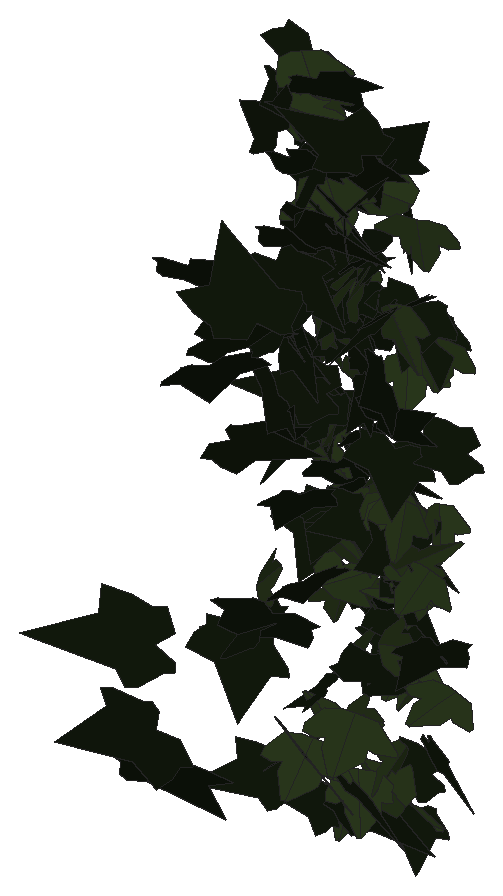
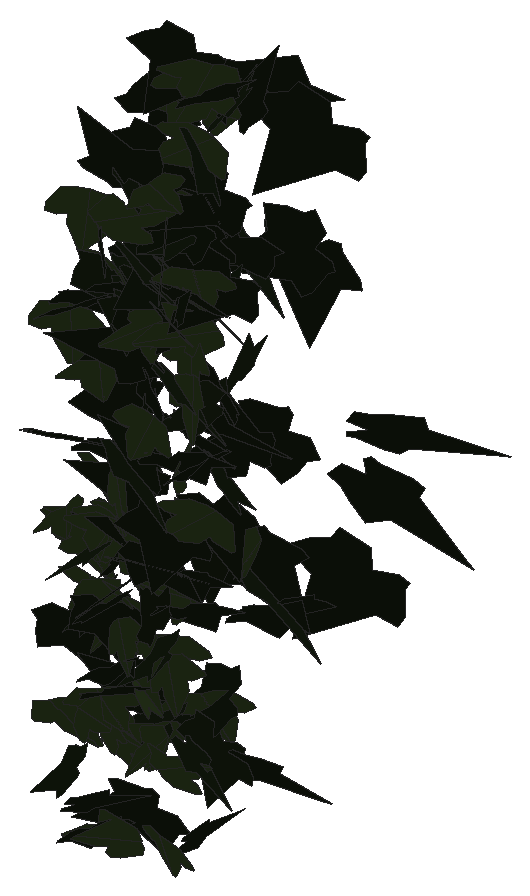
# SketchUp Ruby script. Lengths in inches.
U = 1.inch
M = Sketchup.active_model
def pt(a) = Geom::Point3d.new(a.map { |v| v * U })
def face(e, loops, mat)
  f = e.add_face(loops[0].map { |a| pt(a) })
  loops[1..].each { |l| e.add_face(l.map { |a| pt(a) }).erase! }
  f.material = f.back_material = mat if mat
  f
end
# faces: each face lists its corners as indices into pts; further lists are holes
def faces(e, pts, list, mat = nil) = list.each { |f| face(e, (f[0].is_a?(Array) ? f : [f]).map { |l| l.map { |i| pts[i] } }, mat) }
# xy, xz, yz: faces in a plane at the given z, y or x. An outline is a flat list of corners, or four numbers for a rectangle; further outlines are holes
def ring(l) = l.size == 4 ? [[l[0], l[1]], [l[2], l[1]], [l[2], l[3]], [l[0], l[3]]] : l.each_slice(2).to_a
def flat(e, list, mat, &to3) = list.each { |f| face(e, (f[0].is_a?(Array) ? f : [f]).map { |l| ring(l).map { |u, v| to3.(u, v) } }, mat) }
def xy(e, z, list, mat = nil) = flat(e, list, mat) { |x, y| [x, y, z] }
def xz(e, y, list, mat = nil) = flat(e, list, mat) { |x, z| [x, y, z] }
def yz(e, x, list, mat = nil) = flat(e, list, mat) { |y, z| [x, y, z] }
def lines(e, pts, list) = list.each { |a, b| e.add_line(pt(pts[a]), pt(pts[b])) }
# prism: a flat outline (further loops are holes) pulled along v
def prism(e, loops, v, mat = nil)
  f = face(e, loops, mat); d = Geom::Vector3d.new(v.map { |x| x * U })
  f.pushpull(f.normal.samedirection?(d) ? d.length : -d.length)
end
def box(e, o, s, mat = nil) = prism(e, [[o, [o[0] + s[0], o[1], o[2]], [o[0] + s[0], o[1] + s[1], o[2]], [o[0], o[1] + s[1], o[2]]]], [0, 0, s[2]], mat)
def at(x, y, z, deg = 0) = Geom::Transformation.translation(pt([x, y, z])) * Geom::Transformation.rotation(ORIGIN, Z_AXIS, deg.degrees)
def axes(o, x, y, z) = Geom::Transformation.new([*x, 0, *y, 0, *z, 0, *pt(o).to_a, 1])
def part(name) = M.definitions.add(name)
# library, detail: a bought-in or finely detailed component or shape, given as its bounding box
def library(name, o, s) = part(name).tap { |d| box(d.entities, o, s) }
def detail(e, o, s) = box(e.add_group.entities, o, s)
def put(e, d, t, mat = nil) = e.add_instance(d, t).tap { |i| i.material = mat if mat }
def group(e, t, mat = nil) = e.add_group.tap { |g| g.transformation = t; g.material = mat if mat }.entities
root = M.entities
M.materials.add("1026 AP 7946 SUNNY SIDE UP").color = [254, 231, 186]
M.materials.add("efeu1").color = [18, 25, 13]
M.materials.add("efeu2").color = [43, 57, 29]
c1 = part("ivyleaf_9")
p = [[1.54,2.16,1.25],[1.36,2.04,1.19],[-0.21,0.99,0.68],[-0.71,1.11,0.82],[-0.85,0.86,0.67],[-0.8,0.17,0.21],
  [-0.9,-0.01,0.1],[-0.67,-0.16,-0.02],[-0.08,-0.08,-0.05],[-0.03,-0.6,-0.4],[0.65,-0.88,-0.66],[0.83,-0.6,-0.49],
  [1.29,-0.42,-0.43],[1.8125,-0.07,-0.26],[1.21,0.44,0.15]]
faces(c1.entities,p,[[0,1,2,3,4,5,6,7,8,9,10,11,12,13,14]],"efeu1")
c2 = part("ivyleaf_10")
p = [[0,0.5,-0.03],[-0.0625,2.02,-0.43],[-0.19,2.01,-0.46],[-0.54,1.05,-0.29],[-0.52,0.625,-0.18],[-0.83,0.76,-0.28],
  [-1.16,0.64,-0.33],[-1.15,0.33,-0.24],[-0.77,-0.39,0.02],[-0.3,-0.51,0.16],[0.04,-0.48,0.23],[-0.02,2.01,-0.4375],
  [-0.06,2.01,-0.43],[0.04,-0.49,0.23],[0.67,-0.49,0.14],[1.38,0.36,-0.2],[1.375,0.51,-0.24],[0.81,0.65,-0.19],
  [0.62,0.59,-0.15],[0.6,1.09,-0.28],[0.5,1.23,-0.31]]
faces(c2.entities,p,[[0,1,2,3,4,5,6,7,8,9,10],[11,12,0,13,14,15,16,17,18,19,20]],"efeu2")
put(root,c1,axes([99.1,206.72,271.15],[0.04498,-0.045,-0.44132],[-0.62641,-0.18973,-0.00588],[-0.31896,0.36627,-0.0507]),"1026 AP 7946 SUNNY SIDE UP")
put(root,c1,axes([98.72,207.14,272.19],[-0.51404,0.00428,0.31035],[-0.47955,-0.09831,-0.31579],[0.11029,-0.40748,0.07343]),"1026 AP 7946 SUNNY SIDE UP")
put(root,c1,axes([98.68,207.3,270.18],[0.62161,0.16981,0.02208],[0.03504,-0.00076,-0.43202],[-0.28782,0.36664,-0.00491]),"1026 AP 7946 SUNNY SIDE UP")
put(root,c1,axes([99.86,208,277.3],[-0.67057,-0.05266,0.05626],[0.08156,0.04104,0.42566],[-0.09751,0.39648,-0.0309]),"1026 AP 7946 SUNNY SIDE UP")
put(root,c1,axes([98.4,208.48,277.38],[0.62553,0.17776,0.01998],[0.00654,0.02957,-0.43677],[-0.30296,0.36766,0.03183]),"1026 AP 7946 SUNNY SIDE UP")
put(root,c1,axes([98.43,208.82,275.68],[0.21095,0.37186,-0.04905],[-0.00893,-0.05164,-0.42029],[-0.63702,0.12386,-0.01035]),"1026 AP 7946 SUNNY SIDE UP")
put(root,c1,axes([98.19,209.1,275.91],[0.26985,0.1776,0.31427],[0.39467,0.17871,-0.25004],[-0.42373,0.27956,-0.03275]),"1026 AP 7946 SUNNY SIDE UP")
put(root,c1,axes([98.26,209.78,270.9],[-0.23911,-0.32946,-0.03354],[0.02786,0.02238,-0.38322],[0.56046,-0.14167,0.00474]),"1026 AP 7946 SUNNY SIDE UP")
put(root,c1,axes([98.8,209.67,271.57],[0.1294,0.20948,-0.29899],[-0.33012,-0.21517,-0.23039],[-0.49665,0.1976,0.07524]),"1026 AP 7946 SUNNY SIDE UP")
put(root,c1,axes([99.0625,209.6,276.07],[-0.19036,0.33239,0.11651],[-0.11152,0.08763,-0.37268],[-0.58086,-0.12576,0.03337]),"1026 AP 7946 SUNNY SIDE UP")
put(root,c1,axes([98.55,209.71,271.21],[-0.25067,0.32293,0.10148],[-0.12965,0.064,-0.37665],[-0.55438,-0.16098,0.0422]),"1026 AP 7946 SUNNY SIDE UP")
put(root,c2,axes([99.11,210.09,269.35],[0.4743,0.17614,-0.11601],[-0.12369,-0.0907,-0.35278],[-0.33075,0.28651,-0.03444]),"1026 AP 7946 SUNNY SIDE UP")
put(root,c1,axes([98.78,210.1,269.5],[0.44673,-0.23331,0.02396],[0.00637,-0.034,-0.37619],[0.39834,0.26219,-0.02085]),"1026 AP 7946 SUNNY SIDE UP")
put(root,c2,axes([99.82,210.13,269.97],[0.5272,0.14044,-0.07078],[-0.08561,-0.05286,-0.3645],[-0.25062,0.31349,-0.02437]),"1026 AP 7946 SUNNY SIDE UP")
put(root,c1,axes([98.36,210.375,274.52],[-0.04042,-0.1888,0.29806],[-0.03485,-0.28024,-0.20745],[0.57344,-0.03034,0.0084]),"1026 AP 7946 SUNNY SIDE UP")
put(root,c1,axes([98.49,210.2,268.7],[-0.45262,0.01417,0.14584],[-0.23217,-0.02444,-0.2846],[-0.00247,-0.29833,0.02604]),"1026 AP 7946 SUNNY SIDE UP")
put(root,c2,axes([98.46,209.97,271.8],[0.00956,0.03184,0.33715],[-0.21543,0.28833,-0.02479],[-0.49148,-0.12576,0.01742]),"1026 AP 7946 SUNNY SIDE UP")
put(root,c1,axes([99.05,210.11,271.97],[0.10991,0.33158,0.01218],[0.01766,0.00516,-0.36148],[-0.56272,0.06492,-0.00897]),"1026 AP 7946 SUNNY SIDE UP")
put(root,c1,axes([99.53,210.38,269.03],[0.32232,-0.271,0.0525],[0.0718,-0.03449,-0.35439],[0.46308,0.19397,0.01841]),"1026 AP 7946 SUNNY SIDE UP")
put(root,c1,axes([97.84,210.08,273.76],[0.0256,0.11118,-0.34798],[0.08528,0.32261,0.1246],[0.57924,-0.05241,-0.00297]),"1026 AP 7946 SUNNY SIDE UP")
put(root,c1,axes([98.19,210.56,278.54],[0.06125,0.07775,0.34816],[-0.34612,-0.25285,0.08568],[0.44776,-0.20609,0.01861]),"1026 AP 7946 SUNNY SIDE UP")
put(root,c1,axes([100.32,210.25,275.47],[0.16746,-0.06043,-0.37018],[-0.57964,0.06314,-0.11549],[0.13226,0.35321,-0.03745]),"1026 AP 7946 SUNNY SIDE UP")
put(root,c1,axes([98.41,210.67,275.67],[0.00896,-0.15643,0.2996],[0.01816,-0.28169,-0.1715],[0.54696,0.01192,0.00078]),"1026 AP 7946 SUNNY SIDE UP")
put(root,c1,axes([98.37,210.4,276.58],[-0.09156,-0.13299,-0.32269],[0.25238,0.26077,-0.14889],[0.49606,-0.15722,0.01619]),"1026 AP 7946 SUNNY SIDE UP")
put(root,c2,axes([99.7,210.49,268.87],[0.35392,0.26024,-0.02808],[-0.00632,-0.03491,-0.35691],[-0.44458,0.20767,-0.01728]),"1026 AP 7946 SUNNY SIDE UP")
put(root,c1,axes([98.02,210.59,273.54],[0.2746,0.20994,0.14676],[-0.16858,-0.09261,0.28166],[0.38808,-0.18879,0.01851]),"1026 AP 7946 SUNNY SIDE UP")
put(root,c1,axes([98.625,210.375,269.02],[0.12062,0.28903,0.15336],[0.02741,0.13946,-0.31624],[-0.54409,0.0711,0.01807]),"1026 AP 7946 SUNNY SIDE UP")
put(root,c1,axes([98.05,211.02,278.8],[0.21454,-0.21796,-0.18751],[0.1745,-0.13919,0.26726],[-0.43818,-0.16215,0.01462]),"1026 AP 7946 SUNNY SIDE UP")
put(root,c2,axes([100.21,210.7,268.75],[0.19479,0.04618,0.30215],[-0.4715,0.08782,0.10697],[-0.11132,-0.29115,0.07565]),"1026 AP 7946 SUNNY SIDE UP")
put(root,c2,axes([99.95,211.01,269.17],[0.00722,-0.19655,0.24201],[0.07715,-0.22561,-0.21171],[0.50596,0.03721,0.02883]),"1026 AP 7946 SUNNY SIDE UP")
put(root,c1,axes([99.29,210.97,278.39],[-0.01809,0.0418,0.35658],[-0.5476,-0.0915,-0.00003],[0.15428,-0.31986,0.0417]),"1026 AP 7946 SUNNY SIDE UP")
put(root,c1,axes([98.4,210.82,272.77],[0.09272,0.24876,-0.13909],[-0.05593,-0.12909,-0.27443],[-0.47571,0.06366,0.00515]),"1026 AP 7946 SUNNY SIDE UP")
put(root,c1,axes([98.58,211.12,267.93],[0.02459,-0.21937,-0.16423],[0.07449,-0.14673,0.23138],[-0.44546,-0.03665,0.02963]),"1026 AP 7946 SUNNY SIDE UP")
put(root,c2,axes([98.32,210.88,278.77],[-0.09064,-0.09013,-0.29943],[0.46977,0.07677,-0.08233],[0.16203,-0.273,0.07118]),"1026 AP 7946 SUNNY SIDE UP")
put(root,c1,axes([98.13,211.12,273.54],[-0.32686,0.06498,-0.19825],[0.24268,-0.13294,-0.20998],[-0.23021,-0.2324,0.06013]),"1026 AP 7946 SUNNY SIDE UP")
put(root,c1,axes([98.72,210.85,279.37],[0.43159,0.19588,0.01881],[0.04183,-0.00743,-0.34298],[-0.33087,0.25458,-0.01882]),"1026 AP 7946 SUNNY SIDE UP")
put(root,c1,axes([99.61,211.18,275.9],[-0.36839,0.11376,-0.23066],[0.21062,-0.19885,-0.24729],[-0.35853,-0.2337,0.09173]),"1026 AP 7946 SUNNY SIDE UP")
put(root,c2,axes([98.5,211.03,279.06],[-0.46876,-0.11639,-0.10945],[0.17487,0.01394,-0.31944],[0.19413,-0.2936,0.02347]),"1026 AP 7946 SUNNY SIDE UP")
put(root,c1,axes([98.21,211.03,276.89],[0.42067,-0.03492,0.20078],[0.30703,-0.05702,-0.26738],[0.1053,0.30578,-0.02246]),"1026 AP 7946 SUNNY SIDE UP")
put(root,c2,axes([99.9,211.15,272.89],[0.4863,-0.10978,0.07249],[0.09224,-0.05065,-0.32786],[0.19999,0.29031,-0.02504]),"1026 AP 7946 SUNNY SIDE UP")
put(root,c1,axes([98,211.21,274.88],[-0.08964,-0.08198,-0.28324],[0.46705,-0.03637,-0.04742],[-0.0362,-0.26627,0.08954]),"1026 AP 7946 SUNNY SIDE UP")
put(root,c2,axes([99.82,211.19,275.875],[-0.38142,0.10669,-0.22416],[0.21063,-0.19422,-0.24958],[-0.34125,-0.23913,0.09649]),"1026 AP 7946 SUNNY SIDE UP")
put(root,c2,axes([98.29,211.08,279.37],[0.35467,0.22933,0.0722],[0.09034,0.03862,-0.33129],[-0.39415,0.21521,-0.01097]),"1026 AP 7946 SUNNY SIDE UP")
put(root,c2,axes([98.98,211.25,276.21],[0.069,-0.27403,0.14335],[0.01117,-0.13786,-0.29822],[0.52031,0.0393,-0.01261]),"1026 AP 7946 SUNNY SIDE UP")
put(root,c1,axes([98.5,211.16,274.28],[-0.41855,0.08429,0.19045],[-0.30642,0.01252,-0.27573],[-0.12904,-0.30314,0.037]),"1026 AP 7946 SUNNY SIDE UP")
put(root,c1,axes([99.2,211.07,268.16],[0.00551,-0.01992,-0.31733],[0.36251,0.20585,-0.00944],[0.34994,-0.21293,0.01478]),"1026 AP 7946 SUNNY SIDE UP")
put(root,c1,axes([98.23,211.31,277.75],[-0.31738,0.04031,-0.24954],[0.36565,-0.09537,-0.2035],[-0.16807,-0.28361,0.02848]),"1026 AP 7946 SUNNY SIDE UP")
put(root,c1,axes([99.06,211.4375,274.34],[0.05903,-0.10882,-0.29391],[0.32625,-0.1997,0.10859],[-0.37766,-0.18952,0.04787]),"1026 AP 7946 SUNNY SIDE UP")
put(root,c2,axes([100.17,211.26,271.91],[0.48555,-0.04209,-0.07127],[-0.11474,-0.00653,-0.30914],[0.06709,0.29348,-0.01292]),"1026 AP 7946 SUNNY SIDE UP")
put(root,c1,axes([98.64,211.1,273.9],[-0.42241,0.02151,-0.1385],[-0.21238,0.04624,0.26592],[0.06831,0.27675,-0.02967]),"1026 AP 7946 SUNNY SIDE UP")
put(root,c2,axes([98.72,211.18,271.4],[0.29545,-0.0202,-0.22228],[0.35325,0.03013,0.18426],[0.01738,-0.26904,0.0335]),"1026 AP 7946 SUNNY SIDE UP")
put(root,c1,axes([99.43,211.28,274.11],[0.49815,0.04603,-0.07938],[0.116,0.04396,0.31679],[0.09354,-0.29962,0.02991]),"1026 AP 7946 SUNNY SIDE UP")
put(root,c2,axes([99.1875,211.02,276.03],[0.06679,0.04029,0.34175],[-0.2496,0.28772,-0.01549],[-0.48482,-0.14258,0.05506]),"1026 AP 7946 SUNNY SIDE UP")
put(root,c1,axes([99.57,211.42,273.61],[-0.22894,-0.27039,-0.04499],[0.07744,0.02003,-0.32143],[0.45711,-0.13882,0.03192]),"1026 AP 7946 SUNNY SIDE UP")
put(root,c1,axes([98.8125,211.27,276.37],[-0.45541,0.19917,0.0082],[-0.03407,-0.01856,-0.35681],[-0.33648,-0.26768,0.02503]),"1026 AP 7946 SUNNY SIDE UP")
put(root,c1,axes([98.03,211.5,279.3],[-0.24294,-0.2408,0.12457],[-0.06021,-0.11728,-0.30012],[0.45234,-0.14494,0.02696]),"1026 AP 7946 SUNNY SIDE UP")
put(root,c2,axes([98.79,211.34,267.91],[0.39599,-0.10277,0.05081],[0.05933,-0.04121,-0.27234],[0.18379,0.23473,-0.02156]),"1026 AP 7946 SUNNY SIDE UP")
put(root,c2,axes([99.78,211.05,270.8],[-0.02378,0.12535,0.30025],[-0.10069,0.27269,-0.13064],[-0.50908,-0.05979,0.01181]),"1026 AP 7946 SUNNY SIDE UP")
put(root,c2,axes([98.54,211.26,277.45],[0.44939,0.11956,0.10313],[0.13234,0.05714,-0.30951],[-0.22262,0.27531,0.02419]),"1026 AP 7946 SUNNY SIDE UP")
put(root,c1,axes([98.02,211.18,277.74],[0.55842,0.05066,0.04556],[0.07506,-0.01232,-0.35593],[-0.08258,0.33138,-0.01546]),"1026 AP 7946 SUNNY SIDE UP")
put(root,c2,axes([98.41,211.52,273.6],[-0.0775,0.02247,0.32677],[0.24738,-0.26945,0.04086],[0.4563,0.1499,0.03335]),"1026 AP 7946 SUNNY SIDE UP")
put(root,c2,axes([98.24,211.3,278.43],[-0.38262,-0.02317,-0.20572],[0.3278,-0.03846,-0.23844],[-0.01275,-0.29348,0.0433]),"1026 AP 7946 SUNNY SIDE UP")
put(root,c1,axes([99.46,211.5625,271.92],[-0.13307,-0.11941,0.26483],[-0.17774,-0.22657,-0.15482],[0.43365,-0.12951,0.01781]),"1026 AP 7946 SUNNY SIDE UP")
put(root,c1,axes([98.86,211.22,278.05],[0.50715,0.13258,-0.08467],[-0.10651,-0.05721,-0.34961],[-0.24109,0.30416,-0.02365]),"1026 AP 7946 SUNNY SIDE UP")
put(root,c2,axes([98.76,211.34,269],[0.27331,0.05488,0.21411],[-0.33745,-0.02809,0.17983],[0.09614,-0.25464,0.02254]),"1026 AP 7946 SUNNY SIDE UP")
put(root,c1,axes([98.9,211.57,272.24],[-0.24224,-0.09638,0.22833],[-0.2035,-0.18608,-0.17746],[0.34348,-0.17822,0.05589]),"1026 AP 7946 SUNNY SIDE UP")
put(root,c1,axes([98.25,211.35,277.24],[0.48597,-0.12637,0.00793],[-0.00471,-0.02862,-0.33414],[0.21502,0.28499,-0.02524]),"1026 AP 7946 SUNNY SIDE UP")
put(root,c1,axes([98.39,211.37,277.07],[0.33888,-0.22528,-0.03816],[0.01937,0.05335,-0.3181],[0.38595,0.19513,0.04947]),"1026 AP 7946 SUNNY SIDE UP")
put(root,c1,axes([97.85,211.24,276.53],[0.46895,0.16759,0.0311],[0.07034,-0.01682,-0.34403],[-0.27941,0.27705,-0.03441]),"1026 AP 7946 SUNNY SIDE UP")
put(root,c1,axes([100.29,211.42,270.8],[0.059,0.20528,-0.22659],[-0.03403,-0.21368,-0.22556],[-0.50264,0.03856,-0.01133]),"1026 AP 7946 SUNNY SIDE UP")
put(root,c1,axes([98.68,211.4,275.59],[0.23134,-0.25857,-0.12232],[-0.11049,0.09089,-0.31127],[0.46463,0.15035,-0.01312]),"1026 AP 7946 SUNNY SIDE UP")
put(root,c1,axes([97.97,211.39,274.7],[0.39291,-0.20431,-0.04694],[-0.02107,0.04792,-0.32854],[0.35317,0.23015,0.03262]),"1026 AP 7946 SUNNY SIDE UP")
put(root,c2,axes([99.97,211.28,272.02],[-0.07651,-0.18898,0.25402],[0.1646,0.22093,0.20904],[-0.49137,0.10343,0.03047]),"1026 AP 7946 SUNNY SIDE UP")
put(root,c1,axes([99.73,211.26,275.95],[0.0375,0.32653,0.00975],[-0.02215,0.00574,-0.35],[-0.55391,0.02188,0.01465]),"1026 AP 7946 SUNNY SIDE UP")
put(root,c1,axes([99.32,211.51,277.8125],[-0.3431,0.17537,-0.20052],[0.18114,-0.16252,-0.285],[-0.39923,-0.22445,0.04301]),"1026 AP 7946 SUNNY SIDE UP")
put(root,c1,axes([98.37,211.39,269.49],[-0.22013,0.21481,-0.03444],[0.00984,-0.03729,-0.26871],[-0.36931,-0.12903,0.01337]),"1026 AP 7946 SUNNY SIDE UP")
put(root,c1,axes([99.13,211.3125,269.95],[-0.09111,-0.00249,0.29922],[0.46521,0.05563,0.05764],[-0.09353,0.27914,-0.00477]),"1026 AP 7946 SUNNY SIDE UP")
put(root,c1,axes([98.89,211.55,275.94],[-0.48924,0.05775,-0.14846],[0.21969,-0.06001,-0.31385],[-0.13176,-0.31448,0.02793]),"1026 AP 7946 SUNNY SIDE UP")
put(root,c2,axes([98.37,211.41,275.4],[-0.43038,0.17929,0.08264],[-0.14754,0.00541,-0.32893],[-0.29497,-0.26429,0.04395]),"1026 AP 7946 SUNNY SIDE UP")
put(root,c2,axes([99,211.26,269.27],[-0.02345,0.1072,0.29103],[-0.07489,0.26684,-0.11193],[-0.48813,-0.04609,0.00319]),"1026 AP 7946 SUNNY SIDE UP")
put(root,c1,axes([98.47,211.625,276.29],[-0.45892,-0.10392,-0.07328],[0.12767,-0.01005,-0.30789],[0.16672,-0.27837,0.03404]),"1026 AP 7946 SUNNY SIDE UP")
put(root,c2,axes([98.41,211.57,271.8],[-0.13834,0.03462,-0.26268],[0.34578,-0.13855,-0.09512],[-0.24086,-0.21879,0.01431]),"1026 AP 7946 SUNNY SIDE UP")
put(root,c1,axes([99.8,211.69,275.86],[-0.25873,-0.27533,0.01125],[0.01311,-0.02037,-0.33673],[0.46781,-0.15171,0.01566]),"1026 AP 7946 SUNNY SIDE UP")
put(root,c1,axes([98.02,211.63,273.89],[0.0033,-0.28599,-0.00623],[-0.00049,0.00209,-0.30616],[0.4855,0.00195,-0.00027]),"1026 AP 7946 SUNNY SIDE UP")
put(root,c1,axes([98.81,211.25,276.21],[0.22804,0.18127,0.24447],[0.17701,0.20215,-0.23713],[-0.45882,0.16808,0.03001]),"1026 AP 7946 SUNNY SIDE UP")
put(root,c1,axes([99.22,211.5,276.55],[-0.38458,0.22388,-0.03411],[0.01445,-0.04074,-0.34068],[-0.38434,-0.22556,0.02132]),"1026 AP 7946 SUNNY SIDE UP")
put(root,c1,axes([98.32,211.65,272.18],[-0.33127,-0.17176,-0.04007],[0.07494,0.00282,-0.27679],[0.28803,-0.19827,0.02593]),"1026 AP 7946 SUNNY SIDE UP")
put(root,c1,axes([99.75,211.66,267.93],[-0.12328,-0.26687,-0.00587],[0.00804,0.00079,-0.29605],[0.45296,-0.07265,0.00366]),"1026 AP 7946 SUNNY SIDE UP")
put(root,c2,axes([99.74,211.61,271.54],[0.49517,-0.03637,0.03998],[0.05639,-0.03736,-0.31327],[0.06895,0.29176,-0.03092]),"1026 AP 7946 SUNNY SIDE UP")
put(root,c2,axes([98.91,211.68,270.36],[0.11193,-0.23653,0.14995],[0.05286,-0.13987,-0.26474],[0.46634,0.07263,-0.00598]),"1026 AP 7946 SUNNY SIDE UP")
put(root,c1,axes([98.84,211.45,273.51],[0.15248,0.25846,-0.00707],[-0.03185,0.01704,0.29211],[0.43792,-0.08875,0.0237]),"1026 AP 7946 SUNNY SIDE UP")
put(root,c1,axes([98.88,211.61,273.15],[0.26298,-0.09313,0.24891],[0.32887,-0.13095,-0.19517],[0.27248,0.24794,-0.00467]),"1026 AP 7946 SUNNY SIDE UP")
put(root,c1,axes([98.71,211.43,277.01],[0.14199,-0.08243,-0.3043],[-0.40699,0.15239,-0.12118],[0.29154,0.25289,-0.02097]),"1026 AP 7946 SUNNY SIDE UP")
put(root,c1,axes([99.67,211.59,271.33],[0.25646,-0.23963,-0.08421],[-0.0915,0.05518,-0.30204],[0.41659,0.15964,-0.01449]),"1026 AP 7946 SUNNY SIDE UP")
put(root,c1,axes([98.29,211.73,276.07],[-0.10587,0.04323,0.28463],[-0.04929,-0.27184,0.03632],[0.45364,-0.01945,0.07037]),"1026 AP 7946 SUNNY SIDE UP")
put(root,c1,axes([98.32,211.74,273.95],[-0.36376,-0.21033,-0.01291],[0.04712,-0.01505,-0.32003],[0.35427,-0.21396,0.02931]),"1026 AP 7946 SUNNY SIDE UP")
put(root,c1,axes([98.16,211.34,278.19],[0.02285,0.15643,0.30174],[0.02251,0.27954,-0.1641],[-0.54371,0.01815,0.00589]),"1026 AP 7946 SUNNY SIDE UP")
put(root,c1,axes([99.95,211.77,275.63],[-0.10663,-0.29617,0.01059],[0.06517,-0.02206,-0.32128],[0.49906,-0.0604,0.04422]),"1026 AP 7946 SUNNY SIDE UP")
put(root,c2,axes([100.15,211.64,275.35],[-0.523,-0.0487,0.02701],[-0.02222,-0.07799,-0.32529],[0.09093,-0.29917,0.07584]),"1026 AP 7946 SUNNY SIDE UP")
put(root,c2,axes([99.86,211.61,277.12],[-0.50105,-0.10213,-0.01194],[0.03524,-0.03014,-0.33266],[0.17056,-0.29378,0.03364]),"1026 AP 7946 SUNNY SIDE UP")
put(root,c1,axes([98.09,211.79,271.8125],[-0.32588,-0.22218,0.00881],[0.02799,-0.02887,-0.31296],[0.37659,-0.19011,0.03089]),"1026 AP 7946 SUNNY SIDE UP")
put(root,c1,axes([98.55,211.6,275],[-0.33989,0.20759,-0.01648],[-0.00376,-0.02722,-0.30838],[-0.35372,-0.19919,0.01911]),"1026 AP 7946 SUNNY SIDE UP")
put(root,c2,axes([99.71,211.75,271.38],[0.11366,0.00781,-0.31017],[-0.43429,-0.12187,-0.07227],[-0.18902,0.28469,-0.02046]),"1026 AP 7946 SUNNY SIDE UP")
put(root,c2,axes([98.02,211.68,276.69],[0.4307,0.13891,-0.04662],[-0.05093,-0.03942,-0.30949],[-0.24278,0.25471,-0.01778]),"1026 AP 7946 SUNNY SIDE UP")
put(root,c2,axes([99.28,211.55,267.89],[0.05903,0.05857,0.28987],[0.37231,0.15963,-0.06509],[-0.2852,0.22051,-0.02497]),"1026 AP 7946 SUNNY SIDE UP")
put(root,c2,axes([98.08,211.5,275.78],[0.14209,0.11172,0.31567],[0.32433,0.22282,-0.14607],[-0.42289,0.20843,-0.00596]),"1026 AP 7946 SUNNY SIDE UP")
put(root,c2,axes([99.6,211.69,274.83],[0.30338,0.24473,-0.05769],[-0.03545,-0.05533,-0.32477],[-0.42511,0.17926,-0.01409]),"1026 AP 7946 SUNNY SIDE UP")
put(root,c1,axes([98.67,211.8,274.86],[-0.10885,-0.03031,-0.28288],[0.43765,-0.07222,-0.05921],[-0.10815,-0.26173,0.04512]),"1026 AP 7946 SUNNY SIDE UP")
put(root,c2,axes([99.16,211.76,272.7],[-0.35046,0.06574,-0.18083],[0.18813,-0.15825,-0.2121],[-0.24517,-0.2154,0.09573]),"1026 AP 7946 SUNNY SIDE UP")
put(root,c2,axes([99.4,211.66,272.51],[0.41314,0.15576,0.08333],[0.10905,0.04026,-0.30878],[-0.2731,0.25171,0.00277]),"1026 AP 7946 SUNNY SIDE UP")
put(root,c2,axes([99.35,211.67,272.58],[0.48412,0.04712,0.08325],[0.11589,0.05508,-0.30544],[-0.10059,0.29026,0.04876]),"1026 AP 7946 SUNNY SIDE UP")
put(root,c1,axes([99.64,211.57,272.23],[-0.47422,0.09254,0.01158],[0.02004,0.00509,0.31499],[0.15666,0.27947,-0.00524]),"1026 AP 7946 SUNNY SIDE UP")
put(root,c1,axes([99.55,211.65,272.22],[0.30638,-0.19178,-0.13978],[-0.07459,0.13105,-0.27456],[0.3843,0.17833,0.05815]),"1026 AP 7946 SUNNY SIDE UP")
put(root,c2,axes([98.2,211.59,274.94],[-0.36059,0.19148,0.15732],[-0.21581,0.07374,-0.30376],[-0.34526,-0.24607,0.02556]),"1026 AP 7946 SUNNY SIDE UP")
put(root,c2,axes([97.85,211.72,273.22],[-0.40957,-0.07426,-0.18906],[0.32069,-0.05462,-0.25388],[0.04397,-0.29338,0.09062]),"1026 AP 7946 SUNNY SIDE UP")
put(root,c2,axes([99.27,211.68,273.22],[-0.02133,-0.29237,-0.09091],[-0.00928,0.08138,-0.31202],[0.51497,-0.01064,-0.00939]),"1026 AP 7946 SUNNY SIDE UP")
put(root,c1,axes([98.84,211.65,275.25],[0.28519,0.02617,0.27918],[0.44427,-0.0121,-0.17961],[-0.00674,0.30968,-0.02625]),"1026 AP 7946 SUNNY SIDE UP")
put(root,c1,axes([100.38,211.9,273.66],[-0.44278,0.03862,0.1601],[-0.25469,-0.12962,-0.24695],[0.05871,-0.27101,0.1362]),"1026 AP 7946 SUNNY SIDE UP")
put(root,c1,axes([99.76,211.9375,268.41],[-0.26227,-0.03545,0.22124],[-0.27013,-0.14815,-0.1563],[0.23295,-0.21171,0.06784]),"1026 AP 7946 SUNNY SIDE UP")
put(root,c1,axes([99.4375,211.72,271.32],[0.10838,0.22691,-0.13726],[-0.09459,-0.12017,-0.25327],[-0.43475,0.08272,0.02088]),"1026 AP 7946 SUNNY SIDE UP")
put(root,c1,axes([99.29,211.95,271.64],[-0.00935,-0.28493,0.07481],[-0.01527,-0.0734,-0.30602],[0.49931,-0.00758,-0.00796]),"1026 AP 7946 SUNNY SIDE UP")
put(root,c2,axes([100.07,211.82,272.59],[0.11257,0.26725,-0.10172],[-0.0182,-0.09872,-0.29585],[-0.48315,0.06598,-0.01256]),"1026 AP 7946 SUNNY SIDE UP")
put(root,c1,axes([98.44,211.98,271.52],[0.05664,-0.1391,0.26379],[0.07279,-0.2528,-0.14921],[0.45349,0.05795,-0.00899]),"1026 AP 7946 SUNNY SIDE UP")
put(root,c1,axes([98.94,211.92,272.27],[-0.43437,-0.00061,0.09704],[-0.14009,-0.11075,-0.25174],[0.06367,-0.24784,0.1081]),"1026 AP 7946 SUNNY SIDE UP")
put(root,c2,axes([98.72,211.85,272.36],[0.34869,0.04122,-0.18599],[-0.28375,-0.051,-0.22456],[-0.10905,0.2645,-0.01039]),"1026 AP 7946 SUNNY SIDE UP")
put(root,c1,axes([99.06,211.79,277.89],[-0.2185,-0.00388,0.27692],[0.40669,-0.11094,0.12428],[0.16591,0.26682,0.06006]),"1026 AP 7946 SUNNY SIDE UP")
put(root,c1,axes([99.375,211.85,271.45],[0.0567,-0.26019,-0.09226],[-0.03372,0.0859,-0.26994],[0.4306,0.04099,-0.00899]),"1026 AP 7946 SUNNY SIDE UP")
put(root,c2,axes([99.42,211.86,270.1],[0.40301,0.132,-0.0978],[-0.1219,-0.06195,-0.29102],[-0.24559,0.24736,-0.01604]),"1026 AP 7946 SUNNY SIDE UP")
put(root,c2,axes([99.17,211.9375,277.22],[0.12362,0.12685,0.29777],[-0.27733,-0.22351,0.15273],[0.4356,-0.1783,0.01273]),"1026 AP 7946 SUNNY SIDE UP")
put(root,c1,axes([99.27,211.99,270.26],[-0.28374,-0.18185,0.08101],[-0.02873,-0.08864,-0.26118],[0.33469,-0.16177,0.04625]),"1026 AP 7946 SUNNY SIDE UP")
put(root,c1,axes([98.66,211.88,272.56],[-0.0991,0.16927,-0.21979],[0.00998,-0.21152,-0.18944],[-0.45447,-0.04155,0.04377]),"1026 AP 7946 SUNNY SIDE UP")
put(root,c1,axes([98.41,211.8125,271.0625],[0.30615,-0.20866,-0.08441],[-0.07709,0.06135,-0.29435],[0.36908,0.1859,0.00854]),"1026 AP 7946 SUNNY SIDE UP")
put(root,c2,axes([98.31,211.84,270.88],[-0.14006,-0.27395,-0.00476],[0.02135,-0.00288,-0.30602],[0.46455,-0.08246,0.01263]),"1026 AP 7946 SUNNY SIDE UP")
put(root,c2,axes([98.8,211.62,275.65],[-0.06184,-0.07569,-0.32588],[0.28602,0.25257,-0.08558],[0.44718,-0.17202,0.00968]),"1026 AP 7946 SUNNY SIDE UP")
put(root,c1,axes([98.39,211.68,272.89],[0.30164,0.24316,-0.02705],[-0.00358,-0.03362,-0.32231],[-0.41557,0.17678,-0.01686]),"1026 AP 7946 SUNNY SIDE UP")
put(root,c1,axes([99.87,211.88,268.88],[0.28959,-0.2144,-0.02089],[-0.04492,0.00026,-0.2925],[0.36228,0.17141,-0.01956]),"1026 AP 7946 SUNNY SIDE UP")
put(root,c1,axes([99.2,211.96,270.63],[-0.09211,-0.2556,-0.01636],[0.01396,0.01046,-0.27952],[0.43415,-0.05456,0.00552]),"1026 AP 7946 SUNNY SIDE UP")
put(root,c1,axes([99.31,212.01,276.93],[-0.03273,-0.05112,-0.29591],[0.42775,-0.12445,0.0041],[-0.20891,-0.2468,0.05476]),"1026 AP 7946 SUNNY SIDE UP")
put(root,c1,axes([99.15,211.75,273.68],[-0.21271,0.27345,0.00985],[-0.0102,0.00344,-0.32194],[-0.46418,-0.12538,0.00256]),"1026 AP 7946 SUNNY SIDE UP")
put(root,c2,axes([100.07,211.91,269.71],[0.39443,0.04645,-0.16165],[-0.24766,-0.04267,-0.25399],[-0.10538,0.27413,-0.00811]),"1026 AP 7946 SUNNY SIDE UP")
put(root,c2,axes([98.49,211.95,277.96],[0.21719,0.18068,-0.17296],[-0.15683,-0.13541,-0.23889],[-0.38327,0.1578,-0.00025]),"1026 AP 7946 SUNNY SIDE UP")
put(root,c2,axes([99.52,212.04,269.875],[-0.08946,-0.16937,0.22829],[0.07831,-0.22175,-0.17764],[0.45858,0.00483,0.07487]),"1026 AP 7946 SUNNY SIDE UP")
put(root,c2,axes([98.69,211.85,274.36],[-0.4379,0.1067,-0.06029],[0.07167,-0.04816,-0.29805],[-0.19306,-0.25991,0.02611]),"1026 AP 7946 SUNNY SIDE UP")
put(root,c2,axes([99.08,211.87,271.17],[-0.05205,-0.27318,-0.01864],[0.0078,0.01607,-0.28337],[0.43026,-0.03334,0.00288]),"1026 AP 7946 SUNNY SIDE UP")
